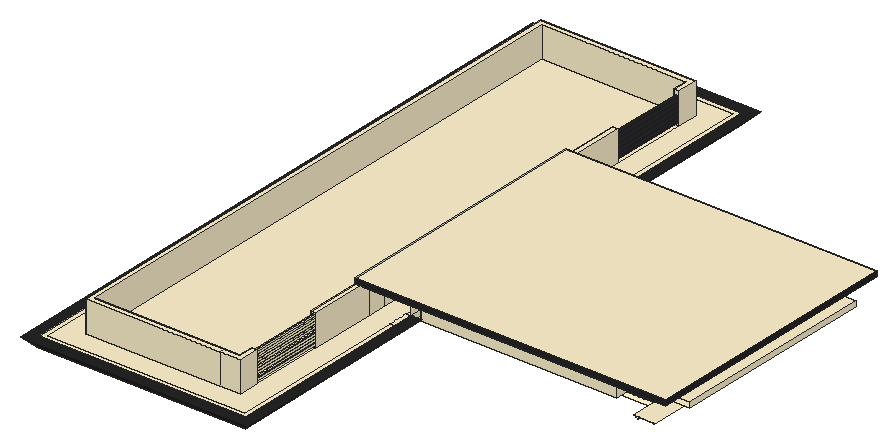
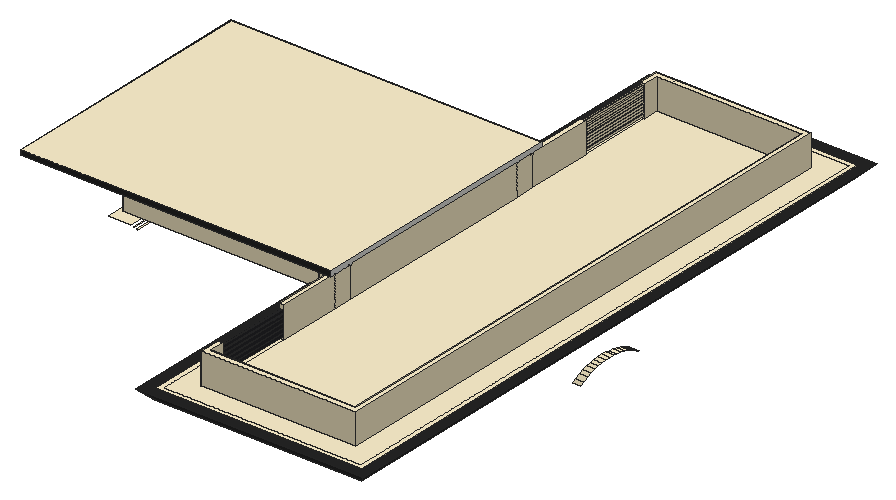
# SketchUp Ruby script. Lengths in inches.
U = 1.inch
M = Sketchup.active_model
def pt(a) = Geom::Point3d.new(a.map { |v| v * U })
def face(e, loops, mat)
  f = e.add_face(loops[0].map { |a| pt(a) })
  loops[1..].each { |l| e.add_face(l.map { |a| pt(a) }).erase! }
  f.material = f.back_material = mat if mat
  f
end
# faces: each face lists its corners as indices into pts; further lists are holes
def faces(e, pts, list, mat = nil) = list.each { |f| face(e, (f[0].is_a?(Array) ? f : [f]).map { |l| l.map { |i| pts[i] } }, mat) }
# xy, xz, yz: faces in a plane at the given z, y or x. An outline is a flat list of corners, or four numbers for a rectangle; further outlines are holes
def ring(l) = l.size == 4 ? [[l[0], l[1]], [l[2], l[1]], [l[2], l[3]], [l[0], l[3]]] : l.each_slice(2).to_a
def flat(e, list, mat, &to3) = list.each { |f| face(e, (f[0].is_a?(Array) ? f : [f]).map { |l| ring(l).map { |u, v| to3.(u, v) } }, mat) }
def xy(e, z, list, mat = nil) = flat(e, list, mat) { |x, y| [x, y, z] }
def xz(e, y, list, mat = nil) = flat(e, list, mat) { |x, z| [x, y, z] }
def yz(e, x, list, mat = nil) = flat(e, list, mat) { |y, z| [x, y, z] }
def lines(e, pts, list) = list.each { |a, b| e.add_line(pt(pts[a]), pt(pts[b])) }
# prism: a flat outline (further loops are holes) pulled along v
def prism(e, loops, v, mat = nil)
  f = face(e, loops, mat); d = Geom::Vector3d.new(v.map { |x| x * U })
  f.pushpull(f.normal.samedirection?(d) ? d.length : -d.length)
end
def box(e, o, s, mat = nil) = prism(e, [[o, [o[0] + s[0], o[1], o[2]], [o[0] + s[0], o[1] + s[1], o[2]], [o[0], o[1] + s[1], o[2]]]], [0, 0, s[2]], mat)
def at(x, y, z, deg = 0) = Geom::Transformation.translation(pt([x, y, z])) * Geom::Transformation.rotation(ORIGIN, Z_AXIS, deg.degrees)
def axes(o, x, y, z) = Geom::Transformation.new([*x, 0, *y, 0, *z, 0, *pt(o).to_a, 1])
def part(name) = M.definitions.add(name)
# library, detail: a bought-in or finely detailed component or shape, given as its bounding box
def library(name, o, s) = part(name).tap { |d| box(d.entities, o, s) }
def detail(e, o, s) = box(e.add_group.entities, o, s)
def put(e, d, t, mat = nil) = e.add_instance(d, t).tap { |i| i.material = mat if mat }
def group(e, t, mat = nil) = e.add_group.tap { |g| g.transformation = t; g.material = mat if mat }.entities
root = M.entities
M.materials.add("Circles_Solid_Black_1K").color = [55, 55, 55]
M.materials.add("D01_Frost_White").color = [255, 242, 206]
M.materials.add("ThomThom - Buttons2").color = [40, 40, 43]
M.materials.add("ThomThom - Hat2").color = [38, 38, 38]
xy(root,358,[[489,290,490,466]],"D01_Frost_White")
xy(root,362,[[490,286,491,470]],"D01_Frost_White")
xy(root,366,[[491,282,516,282.07],[491,282.07,516,474]],"D01_Frost_White")
xy(root,390,[[[12,18,252,258],[18,24,144.65,252]],[[12,258,252,498],[21,264,246,492]],[258,264,486,492],[[12,498,252,738],[18,504,144.65,732]]],"D01_Frost_White")
xy(root,396,[[12,18,252,18,252,234,246,234,246,24,18,24,18,732,246,732,246,258,252,258,252,738,12,738],[[18,24,246,732],[42,48,222,708]],[48,54,216,702],[216,72,222,157.65],[246,234,252,258],
  [216,595.3125,222,684]],"D01_Frost_White")
xy(root,396,[[0,6,264,6,264,258,252,258,252,18,12,18,12,738,252,738,252,498,264,498,264,750,0,750]],"ThomThom - Hat2")
xy(root,397.62,[[218.02,72,220.02,157.65]],"D01_Frost_White")
xy(root,398.39,[[217.9375,595.3125,220.52,684]],"D01_Frost_White")
xy(root,399.62,[[218.02,72,220.02,157.65]],"D01_Frost_White")
xy(root,401.28,[[218.02,72,220.02,157.65]],"D01_Frost_White")
xy(root,401.66,[[217.9375,595.3125,220.52,684]],"ThomThom - Buttons2")
xy(root,403.03,[[217.9375,595.3125,220.52,684]],"ThomThom - Buttons2")
xy(root,403.28,[[218.02,72,220.02,157.65]],"D01_Frost_White")
xy(root,404.89,[[218.02,72,220.02,157.65]],"D01_Frost_White")
xy(root,405,[[516,267,522,489]],"D01_Frost_White")
xy(root,406.3,[[217.9375,595.3125,220.52,684]],"ThomThom - Buttons2")
xy(root,406.89,[[218.02,72,220.02,157.65]],"D01_Frost_White")
xy(root,408.07,[[218.02,72,220.02,157.65]],"D01_Frost_White")
xy(root,408.25,[[217.9375,595.3125,220.52,684]],"ThomThom - Buttons2")
xy(root,410.07,[[218.02,72,220.02,157.65]],"D01_Frost_White")
xy(root,411.53,[[217.9375,595.3125,220.52,684]],"ThomThom - Buttons2")
xy(root,411.57,[[218.02,72,220.02,157.65]],"D01_Frost_White")
xy(root,413.46,[[217.9375,595.3125,220.52,684]],"ThomThom - Buttons2")
xy(root,413.57,[[218.02,72,220.02,157.65]],"D01_Frost_White")
xy(root,414,[[522,258,576,498]],"D01_Frost_White")
xy(root,414.78,[[218.02,72,220.02,157.65]],"D01_Frost_White")
xy(root,416.73,[[217.9375,595.3125,220.52,684]],"ThomThom - Buttons2")
xy(root,416.78,[[218.02,72,220.02,157.65]],"D01_Frost_White")
xy(root,417.71,[[218,72,220,157.65]],"D01_Frost_White")
xy(root,418.5,[[217.9375,595.3125,220.52,684]],"ThomThom - Buttons2")
xy(root,419.71,[[218,72,220,157.65]],"D01_Frost_White")
xy(root,420,[[252,258,540,498]])
xy(root,420,[[540,258,576,498]],"D01_Frost_White")
xy(root,420.42,[[218,72,220,157.65]],"D01_Frost_White")
xy(root,421.77,[[217.9375,595.3125,220.52,684]],"ThomThom - Buttons2")
xy(root,422.42,[[218,72,220,157.65]],"D01_Frost_White")
xy(root,423.04,[[218,72,220,157.65]],"D01_Frost_White")
xy(root,423.53,[[217.9375,595.3125,220.52,684]],"ThomThom - Buttons2")
xy(root,425.04,[[218,72,220,157.65]],"D01_Frost_White")
xy(root,425.57,[[218,72,220,157.65]],"D01_Frost_White")
xy(root,426,[[228,234,564,516]])
xy(root,426,[[[252,258,540,498],[258,264,486,492]]],"D01_Frost_White")
xy(root,426.81,[[217.9375,595.3125,220.52,684]],"ThomThom - Buttons2")
xy(root,427.57,[[218,72,220,157.65]],"D01_Frost_White")
xy(root,428,[[218,72,220,157.65]],"D01_Frost_White")
xy(root,430,[[218,72,220,157.65]],"D01_Frost_White")
xy(root,432,[[216,222,564,234],[564,222,576,528],[216,234,228,516],[228,234,564,516],[216,516,564,528]])
xy(root,432,[[42,48,198,48,198,54,48,54,48,702,216,702,216,684,222,684,222,708,42,708],[198,48,222,48,222,72,216,72,216,54,198,54],[216,157.65,222,595.3125]],"D01_Frost_White")
xy(root,438,[[216,222,576,528]],"D01_Frost_White")
xz(root,18,[[12,384,252,390],[12,390,252,396]],"D01_Frost_White")
xz(root,48,[[42,396,198,432],[198,396,222,432]],"D01_Frost_White")
xz(root,54,[[48,396,216,432]],"D01_Frost_White")
xz(root,72,[[[216,396,222,432],[218.02,397.62,220.02,399.62],[218.02,401.28,220.02,403.28],[218.02,404.89,220.02,406.89],[218.02,408.07,220.02,410.07],[218.02,411.57,220.02,413.57],[218.02,414.78,220.02,416.78],[218,417.71,220,419.71],[218,420.42,220,422.42],[218,423.04,220,425.04],[218,425.57,220,427.57],[218,428,220,430]]],"D01_Frost_White")
xz(root,157.65,[[[216,396,222,432],[218.02,397.62,220.02,399.62],[218.02,401.28,220.02,403.28],[218.02,404.89,220.02,406.89],[218.02,408.07,220.02,410.07],[218.02,411.57,220.02,413.57],[218.02,414.78,220.02,416.78],[218,417.71,220,419.71],[218,420.42,220,422.42],[218,423.04,220,425.04],[218,425.57,220,427.57],[218,428,220,430]]],"D01_Frost_White")
xz(root,222,[[216,432,576,438]],"ThomThom - Hat2")
xz(root,234,[[228,426,564,432]])
xz(root,258,[[252,384,263.99,395.99,258.49,396,252,396],[252,396,258.49,396,252,396.02]],"D01_Frost_White")
xz(root,264,[[258,390,486,426]],"D01_Frost_White")
xz(root,492,[[258,390,486,426]],"D01_Frost_White")
xz(root,516,[[228,426,564,432]])
xz(root,528,[[216,432,576,438]],"ThomThom - Hat2")
xz(root,595.3125,[[[216,396,222,432],[217.9375,398.39,220.52,401.66],[217.9375,403.03,220.52,406.3],[217.9375,408.25,220.52,411.53],[217.9375,413.46,220.52,416.73],[217.9375,418.5,220.52,421.77],[217.9375,423.53,220.52,426.81]]],"D01_Frost_White")
xz(root,684,[[[216,396,222,432],[217.9375,423.53,220.52,426.81],[217.9375,418.5,220.52,421.77],[217.9375,413.46,220.52,416.73],[217.9375,408.25,220.52,411.53],[217.9375,403.03,220.52,406.3],[217.9375,398.39,220.52,401.66]]],"D01_Frost_White")
xz(root,702,[[48,396,216,432]],"D01_Frost_White")
xz(root,708,[[42,396,222,432]],"D01_Frost_White")
xz(root,738,[[12,384,252,390]],"D01_Frost_White")
xz(root,738,[[12,390,252,396]],"ThomThom - Hat2")
yz(root,12,[[18,384,738,390],[18,390,738,396]],"D01_Frost_White")
yz(root,42,[[48,396,708,432]],"D01_Frost_White")
yz(root,48,[[54,396,702,432]],"D01_Frost_White")
yz(root,216,[[222,432,528,438]])
yz(root,216,[[54,396,72,432],[157.65,396,234,432],[234,396,258,432],[258,396,498,432],[498,396,522,432],
  [522,396,595.3125,432],[684,396,702,432]],"D01_Frost_White")
yz(root,217.9375,[[595.3125,398.39,684,401.66],[595.3125,403.03,684,406.3],[595.3125,408.25,684,411.53],[595.3125,413.46,684,416.73],[595.3125,418.5,684,421.77],
  [595.3125,423.53,684,426.81]],"ThomThom - Buttons2")
yz(root,218,[[72,417.71,157.65,419.71],[72,420.42,157.65,422.42],[72,423.04,157.65,425.04],[72,425.57,157.65,427.57],[72,428,157.65,430]],"D01_Frost_White")
yz(root,218.02,[[72,397.62,157.65,399.62],[72,401.28,157.65,403.28],[72,404.89,157.65,406.89],[72,408.07,157.65,410.07],[72,411.57,157.65,413.57],
  [72,414.78,157.65,416.78]],"D01_Frost_White")
yz(root,220,[[72,417.71,157.65,419.71],[72,420.42,157.65,422.42],[72,423.04,157.65,425.04],[72,425.57,157.65,427.57],[72,428,157.65,430]],"D01_Frost_White")
yz(root,220.02,[[72,397.62,157.65,399.62],[72,401.28,157.65,403.28],[72,404.89,157.65,406.89],[72,408.07,157.65,410.07],[72,411.57,157.65,413.57],
  [72,414.78,157.65,416.78]],"D01_Frost_White")
yz(root,220.52,[[595.3125,398.39,684,401.66],[595.3125,403.03,684,406.3],[595.3125,408.25,684,411.53],[595.3125,413.46,684,416.73],[595.3125,418.5,684,421.77],
  [595.3125,423.53,684,426.81]],"ThomThom - Buttons2")
yz(root,222,[[48,396,72,432],[157.65,396,234,432],[234,396,258,432],[258,396,595.3125,432],[684,396,708,432]],"D01_Frost_White")
yz(root,228,[[234,426,516,432]])
yz(root,252,[[18,384,258,390],[498,384,738,390],[258,390,498,396],[258,396,498,426]],"D01_Frost_White")
yz(root,252,[[18,390,258,396],[498,390,738,396]],"ThomThom - Hat2")
yz(root,258,[[264,390,492,426]],"D01_Frost_White")
yz(root,486,[[264,390,492,426]],"D01_Frost_White")
yz(root,489,[[377,353.97,378,354,377,354],[379,353.97,379,354,378,354]],"Circles_Solid_Black_1K")
yz(root,540,[[258,420,498,426]],"D01_Frost_White")
yz(root,564,[[234,426,516,432]])
yz(root,576,[[258,414,498,420]],"D01_Frost_White")
yz(root,576,[[222,432,528,438]],"ThomThom - Hat2")
p = [[21,340.6875,345.28],[21,335.82,342.67],[12,335.82,342.67],[12,340.6875,345.28],[258,340.6875,345.28],[258,335.82,342.67],
  [246,335.82,342.67],[246,340.6875,345.28],[486,340.6875,345.28],[486,335.82,342.67],[489,340.6875,345.28],[489,335.82,342.67],
  [21,420.18,342.67],[21,415.3125,345.28],[12,415.3125,345.28],[12,420.18,342.67],[258,420.18,342.67],[258,415.3125,345.28],
  [246,415.3125,345.28],[246,420.18,342.67],[486,420.18,342.67],[486,415.3125,345.28],[489,420.18,342.67],[489,415.3125,345.28],
  [21,345.71,347.5625],[12,345.71,347.5625],[258,345.71,347.5625],[246,345.71,347.5625],[486,345.71,347.5625],[489,345.71,347.5625],
  [21,410.29,347.5625],[12,410.29,347.5625],[258,410.29,347.5625],[246,410.29,347.5625],[486,410.29,347.5625],[489,410.29,347.5625],
  [21,350.88,349.51],[12,350.88,349.51],[258,350.88,349.51],[246,350.88,349.51],[486,350.88,349.51],[489,350.88,349.51],
  [21,405.12,349.51],[12,405.12,349.51],[258,405.12,349.51],[246,405.12,349.51],[486,405.12,349.51],[489,405.12,349.51],
  [21,356.16,351.12],[12,356.16,351.12],[258,356.16,351.12],[246,356.16,351.12],[486,356.16,351.12],[489,356.16,351.12],
  [21,399.84,351.12],[12,399.84,351.12],[258,399.84,351.12],[246,399.84,351.12],[486,399.84,351.12],[489,399.84,351.12],
  [21,361.54,352.375],[12,361.54,352.375],[258,361.54,352.375],[246,361.54,352.375],[486,361.54,352.375],[489,361.54,352.375],
  [21,394.46,352.375],[12,394.46,352.375],[258,394.46,352.375],[246,394.46,352.375],[486,394.46,352.375],[489,394.46,352.375],
  [21,366.99,353.28],[12,366.99,353.28],[258,366.99,353.28],[246,366.99,353.28],[486,366.99,353.28],[489,366.99,353.28],
  [21,389.01,353.28],[12,389.01,353.28],[258,389.01,353.28],[246,389.01,353.28],[486,389.01,353.28],[489,389.01,353.28],
  [21,372.48,353.82],[12,372.48,353.82],[258,372.48,353.82],[246,372.48,353.82],[486,372.48,353.82],[489,372.48,353.82],
  [21,383.52,353.82],[12,383.52,353.82],[258,383.52,353.82],[246,383.52,353.82],[486,383.52,353.82],[489,383.52,353.82],
  [21,378,354],[12,378,354],[258,378,354],[246,378,354],[486,378,354],[489,377,353.97],
  [489,378,354],[489,379,353.97],[252,18,384],[264,6,396],[0,6,396],[12,18,384],
  [0,750,396],[12,738,384],[252,258,384],[263.99,258,395.99],[264,258,396],[252,498,384],
  [252,738,384],[264,750,396],[264,498,396],[252,498,420],[252,258,420],[228,234,426],
  [228,516,426],[540,258,420],[564,234,426],[540,498,420],[564,516,426],[216,222,432],
  [216,234,432],[216,516,432],[216,528,432],[576,222,432],[564,222,432],[576,528,432],
  [564,528,432],[264,258,395.99],[491.59,474,365.9],[516,474,365.9]]
faces(root,p,[[0,1,2,3],[4,5,6,7],[8,9,5,4],[10,11,9,8],[12,13,14,15],[16,17,18,19],[20,21,17,16],[22,23,21,20],
  [24,0,3,25],[26,4,7,27],[28,8,4,26],[29,10,8,28],[13,30,31,14],[17,32,33,18],[21,34,32,17],[23,35,34,21],
  [36,24,25,37],[38,26,27,39],[40,28,26,38],[41,29,28,40],[30,42,43,31],[32,44,45,33],[34,46,44,32],[35,47,46,34],
  [48,36,37,49],[50,38,39,51],[52,40,38,50],[53,41,40,52],[42,54,55,43],[44,56,57,45],[46,58,56,44],[47,59,58,46],
  [60,48,49,61],[62,50,51,63],[64,52,50,62],[65,53,52,64],[54,66,67,55],[56,68,69,57],[58,70,68,56],[59,71,70,58],
  [72,60,61,73],[74,62,63,75],[76,64,62,74],[77,65,64,76],[66,78,79,67],[68,80,81,69],[70,82,80,68],[71,83,82,70],
  [84,72,73,85],[86,74,75,87],[88,76,74,86],[89,77,76,88],[78,90,91,79],[80,92,93,81],[82,94,92,80],[83,95,94,82],
  [96,84,85,97],[98,86,87,99],[100,88,86,98],[101,89,88,100,102],[90,96,97,91],[92,98,99,93],[94,100,98,92],[103,102,100,94,95]],"D01_Frost_White")
faces(root,p,[[104,105,106,107],[106,108,109,107],[105,104,110,111,112],[113,114,115,116],[114,109,108,115],[119,118,121,122],[122,121,123,124],[124,123,117,120],
  [125,119,122,129,130],[124,131,129,122],[120,128,132,131,124]],"ThomThom - Hat2")
faces(root,p,[[117,118,119,120],[119,125,126,127,128,120]])
lines(root,p,[[111,133],[134,135]])
